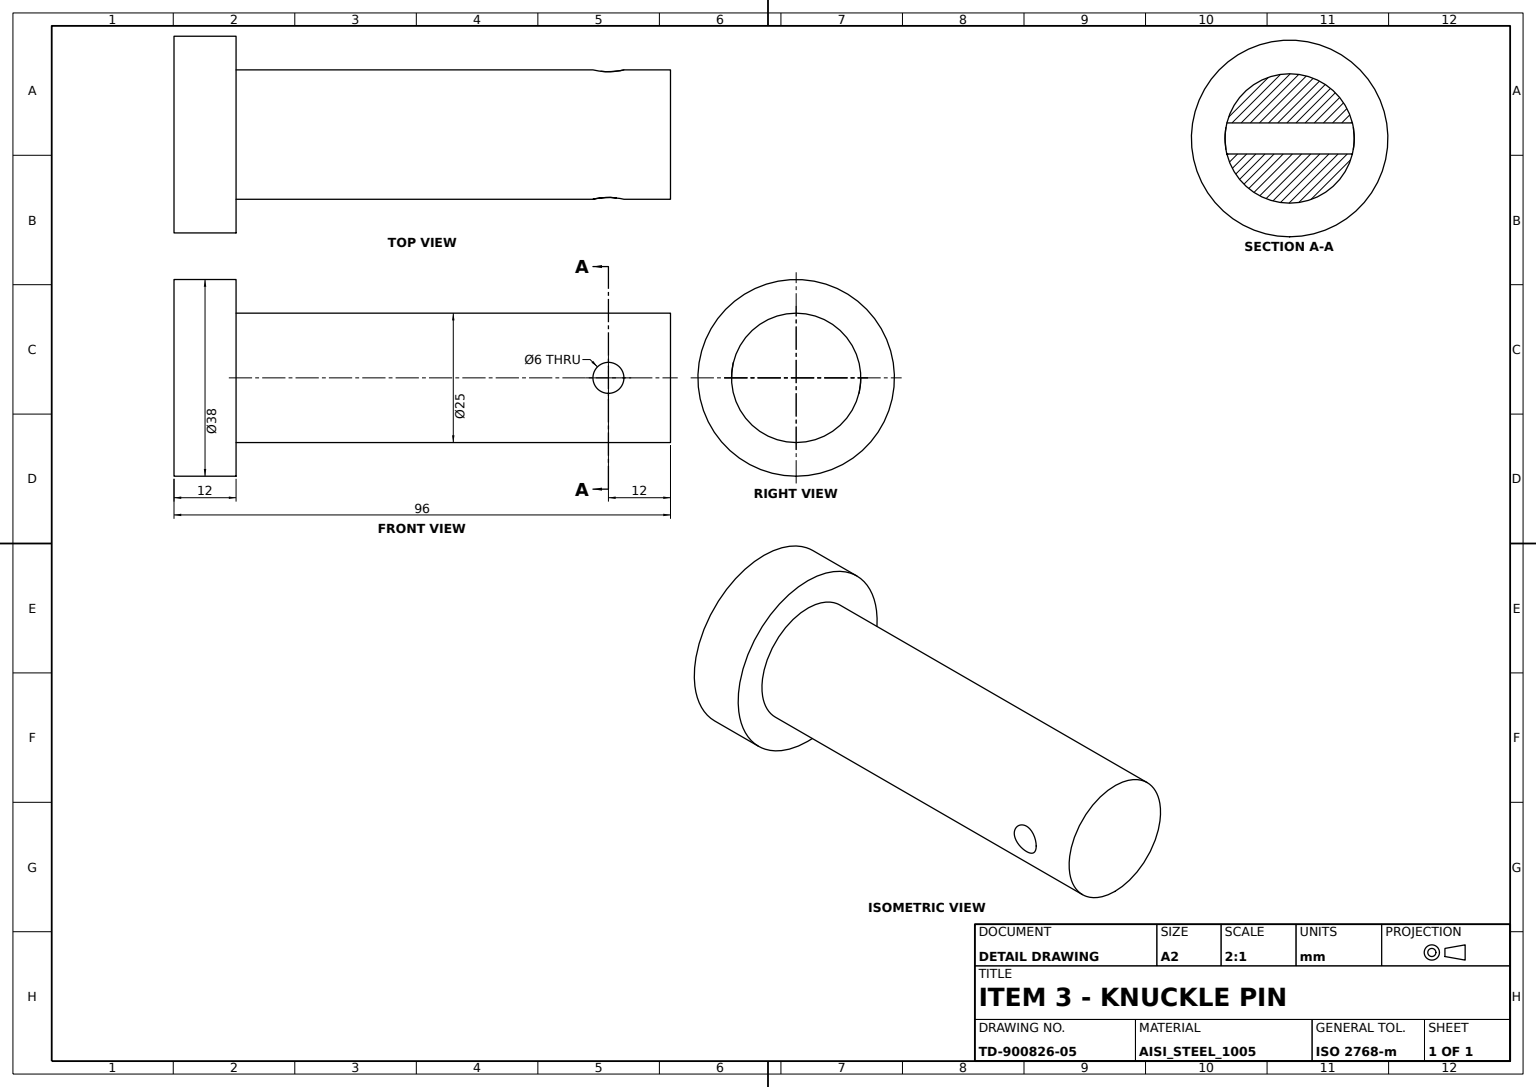
ISO-10303-21;
HEADER;
FILE_DESCRIPTION((''),'2;1');
FILE_NAME('','',(''),(''),'','','');
FILE_SCHEMA(('AUTOMOTIVE_DESIGN'));
ENDSEC;
DATA;
#1=APPLICATION_CONTEXT('');
#2=PRODUCT_CONTEXT('',#1,'mechanical');
#3=PRODUCT('','','',(#2));
#4=PRODUCT_DEFINITION_FORMATION('','',#3);
#5=PRODUCT_DEFINITION_CONTEXT('',#1,'design');
#6=PRODUCT_DEFINITION('','',#4,#5);
#7=PRODUCT_DEFINITION_SHAPE('','',#6);
#8=(LENGTH_UNIT()NAMED_UNIT(*)SI_UNIT(.MILLI.,.METRE.));
#9=(NAMED_UNIT(*)PLANE_ANGLE_UNIT()SI_UNIT($,.RADIAN.));
#10=(NAMED_UNIT(*)SI_UNIT($,.STERADIAN.)SOLID_ANGLE_UNIT());
#11=UNCERTAINTY_MEASURE_WITH_UNIT(LENGTH_MEASURE(0.005),#8,'distance_accuracy_value','');
#12=(GEOMETRIC_REPRESENTATION_CONTEXT(3)GLOBAL_UNCERTAINTY_ASSIGNED_CONTEXT((#11))GLOBAL_UNIT_ASSIGNED_CONTEXT((#8,#9,#10))REPRESENTATION_CONTEXT('',''));
#13=CARTESIAN_POINT('',(0.,-12.5,87.));
#14=VERTEX_POINT('',#13);
#15=CARTESIAN_POINT('',(2.353177,-12.319625,86.348756));
#16=CARTESIAN_POINT('',(-0.000455,-12.590122,87.325521));
#17=CARTESIAN_POINT('',(-2.351355,-12.319889,86.34916));
#18=CARTESIAN_POINT('',(-3.324427,-12.042024,84.003381));
#19=CARTESIAN_POINT('',(-2.350934,-12.319982,81.64854));
#20=CARTESIAN_POINT('',(-0.001353,-12.589884,80.676129));
#21=CARTESIAN_POINT('',(2.34878,-12.32048,81.646945));
#22=CARTESIAN_POINT('',(3.32451,-12.041966,83.998531));
#23=B_SPLINE_CURVE_WITH_KNOTS('',3,(#15,#16,#17,#18,#19,#20,#21,#22,#15,#16,#17),.UNSPECIFIED.,.T.,.F.,(1,1,1,1,1,1,1,1,1,1,1,1,1,1,1),(-0.007059428,-0.004706285,-0.002353143,0.,0.002353143,0.004706285,0.007059428,0.009412571,0.011765714,0.014118856,0.016471999,0.018825142,0.021178284,0.023531427,0.02588457),.UNSPECIFIED.);
#24=EDGE_CURVE('',#14,#14,#23,.T.);
#25=ORIENTED_EDGE('',*,*,#24,.T.);
#26=EDGE_LOOP('',(#25));
#27=FACE_BOUND('',#26,.T.);
#28=CARTESIAN_POINT('',(0.,12.5,87.));
#29=VERTEX_POINT('',#28);
#30=CARTESIAN_POINT('',(-2.353177,12.319625,86.348756));
#31=CARTESIAN_POINT('',(0.000455,12.590122,87.325521));
#32=CARTESIAN_POINT('',(2.351355,12.319889,86.34916));
#33=CARTESIAN_POINT('',(3.324427,12.042024,84.003381));
#34=CARTESIAN_POINT('',(2.350934,12.319982,81.64854));
#35=CARTESIAN_POINT('',(0.001353,12.589884,80.676129));
#36=CARTESIAN_POINT('',(-2.34878,12.32048,81.646945));
#37=CARTESIAN_POINT('',(-3.32451,12.041966,83.998531));
#38=B_SPLINE_CURVE_WITH_KNOTS('',3,(#30,#31,#32,#33,#34,#35,#36,#37,#30,#31,#32),.UNSPECIFIED.,.T.,.F.,(1,1,1,1,1,1,1,1,1,1,1,1,1,1,1),(-0.007059428,-0.004706285,-0.002353143,0.,0.002353143,0.004706285,0.007059428,0.009412571,0.011765714,0.014118856,0.016471999,0.018825142,0.021178284,0.023531427,0.02588457),.UNSPECIFIED.);
#39=EDGE_CURVE('',#29,#29,#38,.T.);
#40=ORIENTED_EDGE('',*,*,#39,.T.);
#41=EDGE_LOOP('',(#40));
#42=FACE_BOUND('',#41,.T.);
#43=CARTESIAN_POINT('',(0.,-55000.,84.));
#44=DIRECTION('',(0.,1.,0.));
#45=DIRECTION('',(0.,0.,1.));
#46=AXIS2_PLACEMENT_3D('',#43,#44,#45);
#47=CYLINDRICAL_SURFACE('',#46,3.);
#48=ADVANCED_FACE('',(#27,#42),#47,.F.);
#49=CARTESIAN_POINT('',(19.,0.,0.));
#50=VERTEX_POINT('',#49);
#51=CARTESIAN_POINT('',(0.,0.,0.));
#52=DIRECTION('',(0.,0.,-1.));
#53=DIRECTION('',(1.,0.,0.));
#54=AXIS2_PLACEMENT_3D('',#51,#52,#53);
#55=CIRCLE('',#54,19.);
#56=EDGE_CURVE('',#50,#50,#55,.T.);
#57=ORIENTED_EDGE('',*,*,#56,.T.);
#58=EDGE_LOOP('',(#57));
#59=FACE_BOUND('',#58,.T.);
#60=DIRECTION('',(-1.,0.,0.));
#61=AXIS2_PLACEMENT_3D('',#51,#52,#60);
#62=PLANE('',#61);
#63=ADVANCED_FACE('',(#59),#62,.T.);
#64=ORIENTED_EDGE('',*,*,#56,.F.);
#65=EDGE_LOOP('',(#64));
#66=FACE_BOUND('',#65,.T.);
#67=CARTESIAN_POINT('',(19.,0.,12.));
#68=VERTEX_POINT('',#67);
#69=CARTESIAN_POINT('',(0.,0.,12.));
#70=AXIS2_PLACEMENT_3D('',#69,#52,#53);
#71=CIRCLE('',#70,19.);
#72=EDGE_CURVE('',#68,#68,#71,.T.);
#73=ORIENTED_EDGE('',*,*,#72,.T.);
#74=EDGE_LOOP('',(#73));
#75=FACE_BOUND('',#74,.T.);
#76=AXIS2_PLACEMENT_3D('',#69,#52,#60);
#77=CYLINDRICAL_SURFACE('',#76,19.);
#78=ADVANCED_FACE('',(#66,#75),#77,.T.);
#79=CARTESIAN_POINT('',(12.5,0.,96.));
#80=VERTEX_POINT('',#79);
#81=CARTESIAN_POINT('',(0.,0.,96.));
#82=AXIS2_PLACEMENT_3D('',#81,#52,#53);
#83=CIRCLE('',#82,12.5);
#84=EDGE_CURVE('',#80,#80,#83,.T.);
#85=ORIENTED_EDGE('',*,*,#84,.T.);
#86=EDGE_LOOP('',(#85));
#87=FACE_BOUND('',#86,.T.);
#88=CARTESIAN_POINT('',(12.5,0.,12.));
#89=VERTEX_POINT('',#88);
#90=CIRCLE('',#70,12.5);
#91=EDGE_CURVE('',#89,#89,#90,.T.);
#92=ORIENTED_EDGE('',*,*,#91,.F.);
#93=EDGE_LOOP('',(#92));
#94=FACE_BOUND('',#93,.T.);
#95=ORIENTED_EDGE('',*,*,#24,.F.);
#96=EDGE_LOOP('',(#95));
#97=FACE_BOUND('',#96,.T.);
#98=ORIENTED_EDGE('',*,*,#39,.F.);
#99=EDGE_LOOP('',(#98));
#100=FACE_BOUND('',#99,.T.);
#101=AXIS2_PLACEMENT_3D('',#81,#52,#60);
#102=CYLINDRICAL_SURFACE('',#101,12.5);
#103=ADVANCED_FACE('',(#87,#94,#97,#100),#102,.T.);
#104=ORIENTED_EDGE('',*,*,#72,.F.);
#105=EDGE_LOOP('',(#104));
#106=FACE_BOUND('',#105,.T.);
#107=ORIENTED_EDGE('',*,*,#91,.T.);
#108=EDGE_LOOP('',(#107));
#109=FACE_BOUND('',#108,.T.);
#110=PLANE('',#76);
#111=ADVANCED_FACE('',(#106,#109),#110,.F.);
#112=ORIENTED_EDGE('',*,*,#84,.F.);
#113=EDGE_LOOP('',(#112));
#114=FACE_BOUND('',#113,.T.);
#115=PLANE('',#101);
#116=ADVANCED_FACE('',(#114),#115,.F.);
#117=CLOSED_SHELL('',(#48,#63,#78,#103,#111,#116));
#118=MANIFOLD_SOLID_BREP('',#117);
#119=ADVANCED_BREP_SHAPE_REPRESENTATION('',(#118),#12);
#120=SHAPE_DEFINITION_REPRESENTATION(#7,#119);
ENDSEC;
END-ISO-10303-21;
